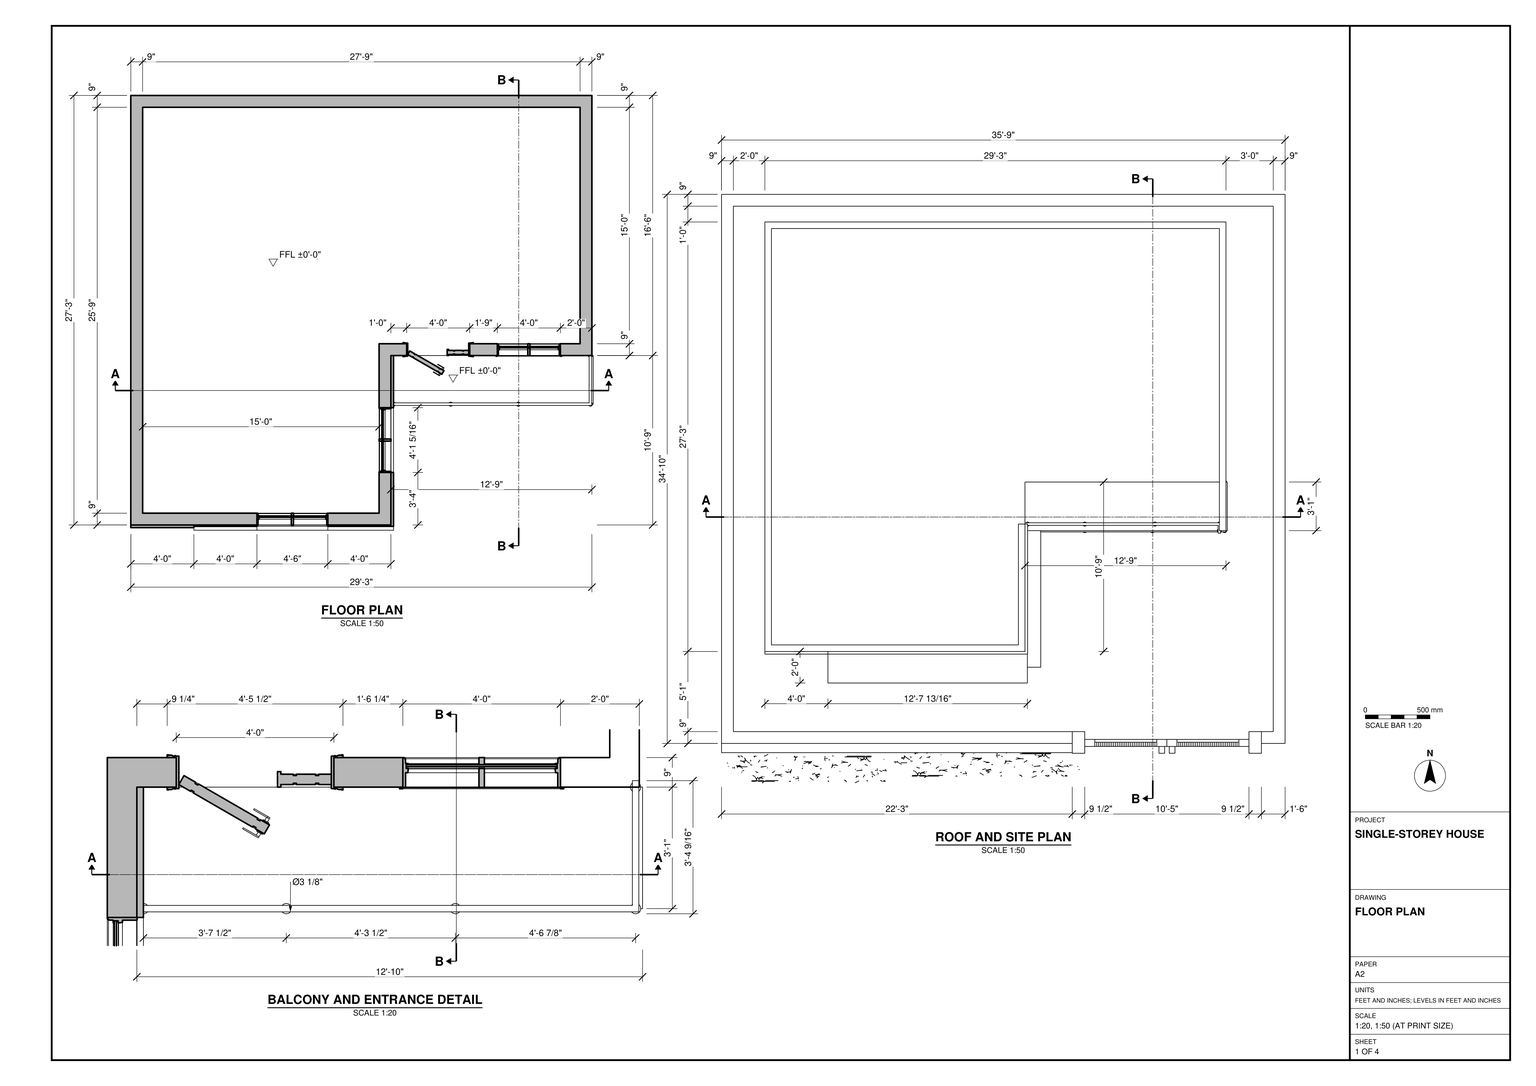
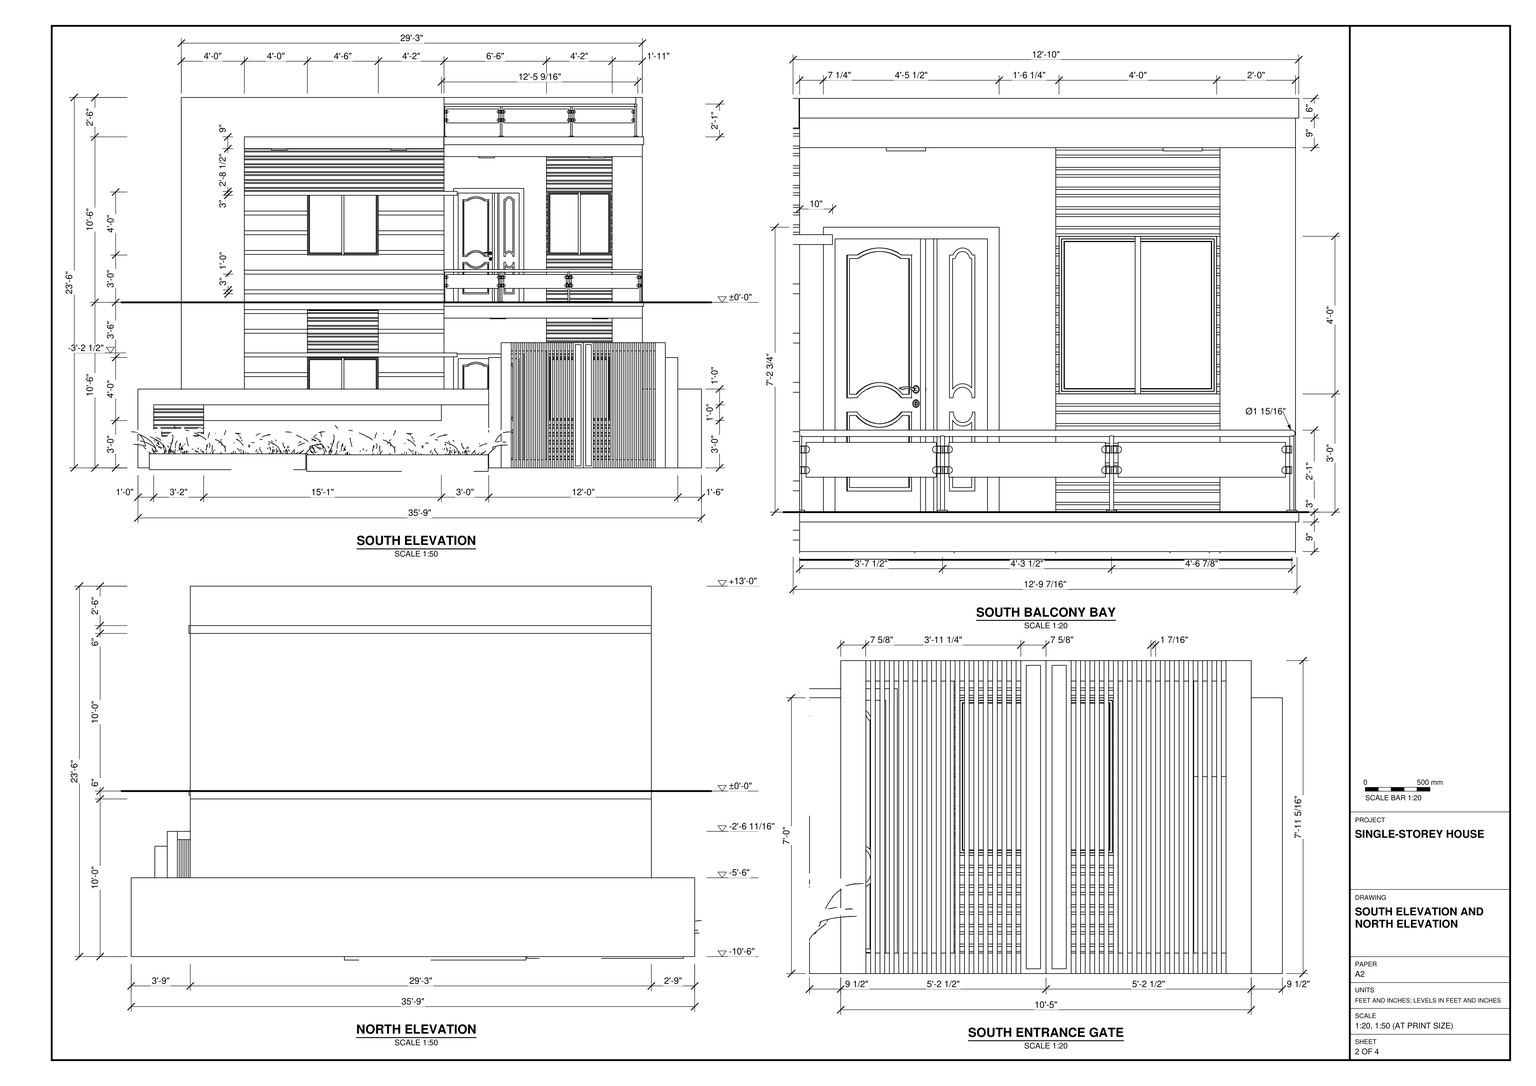
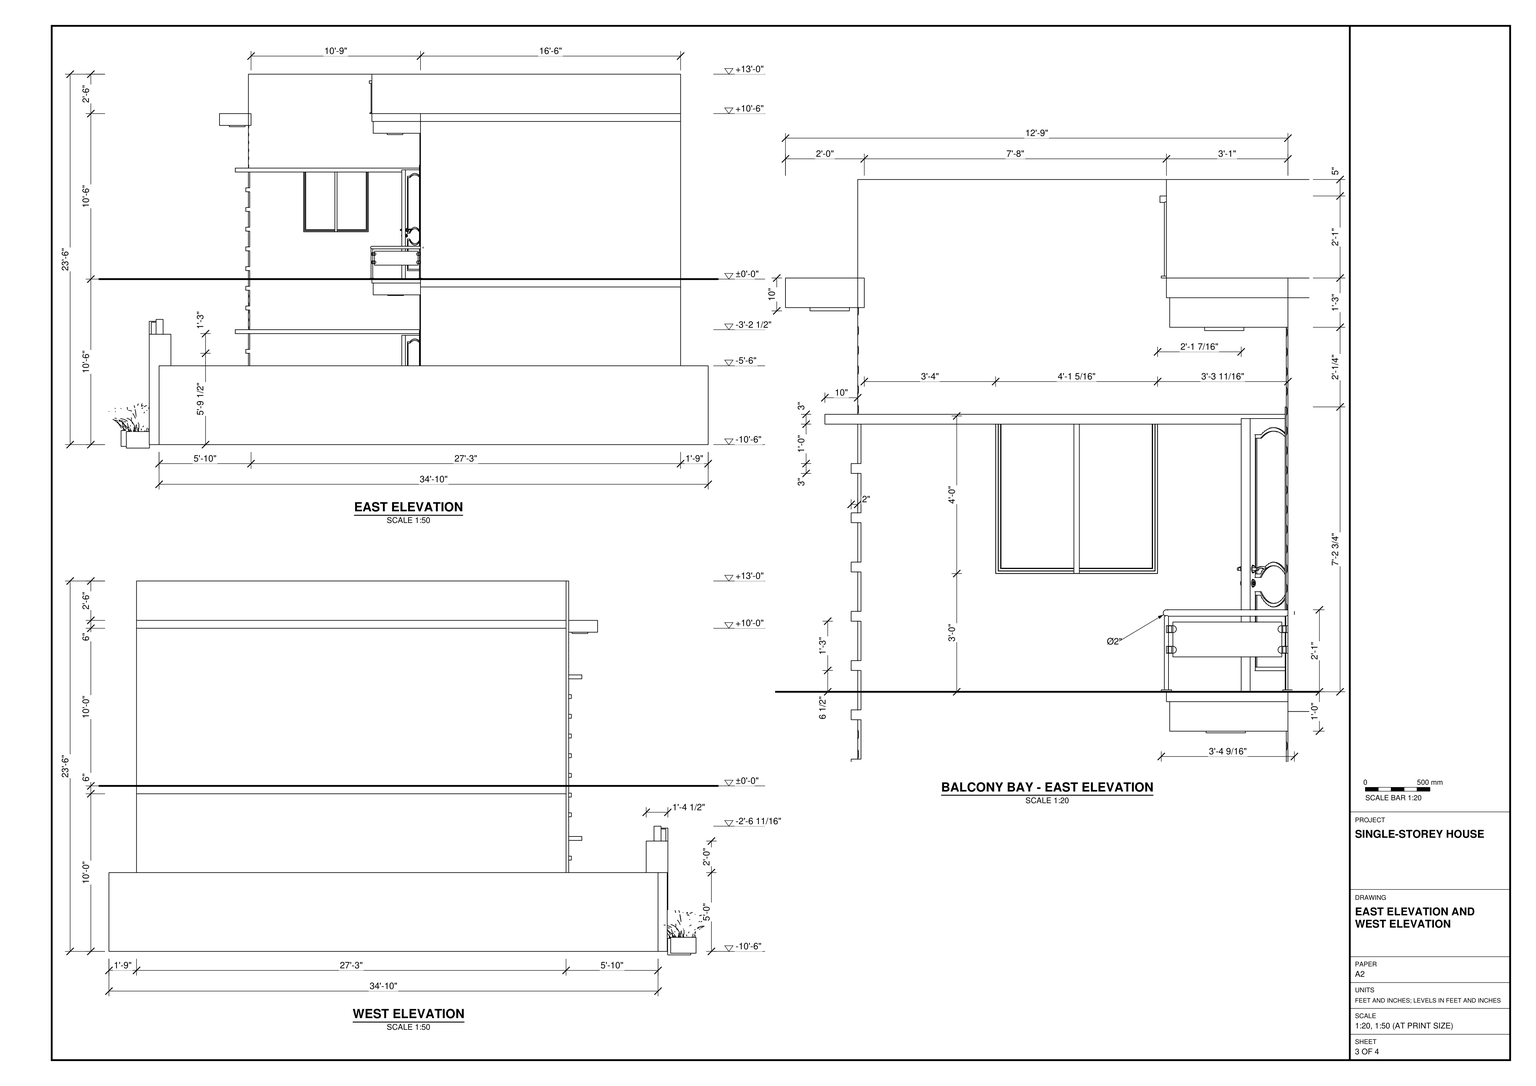
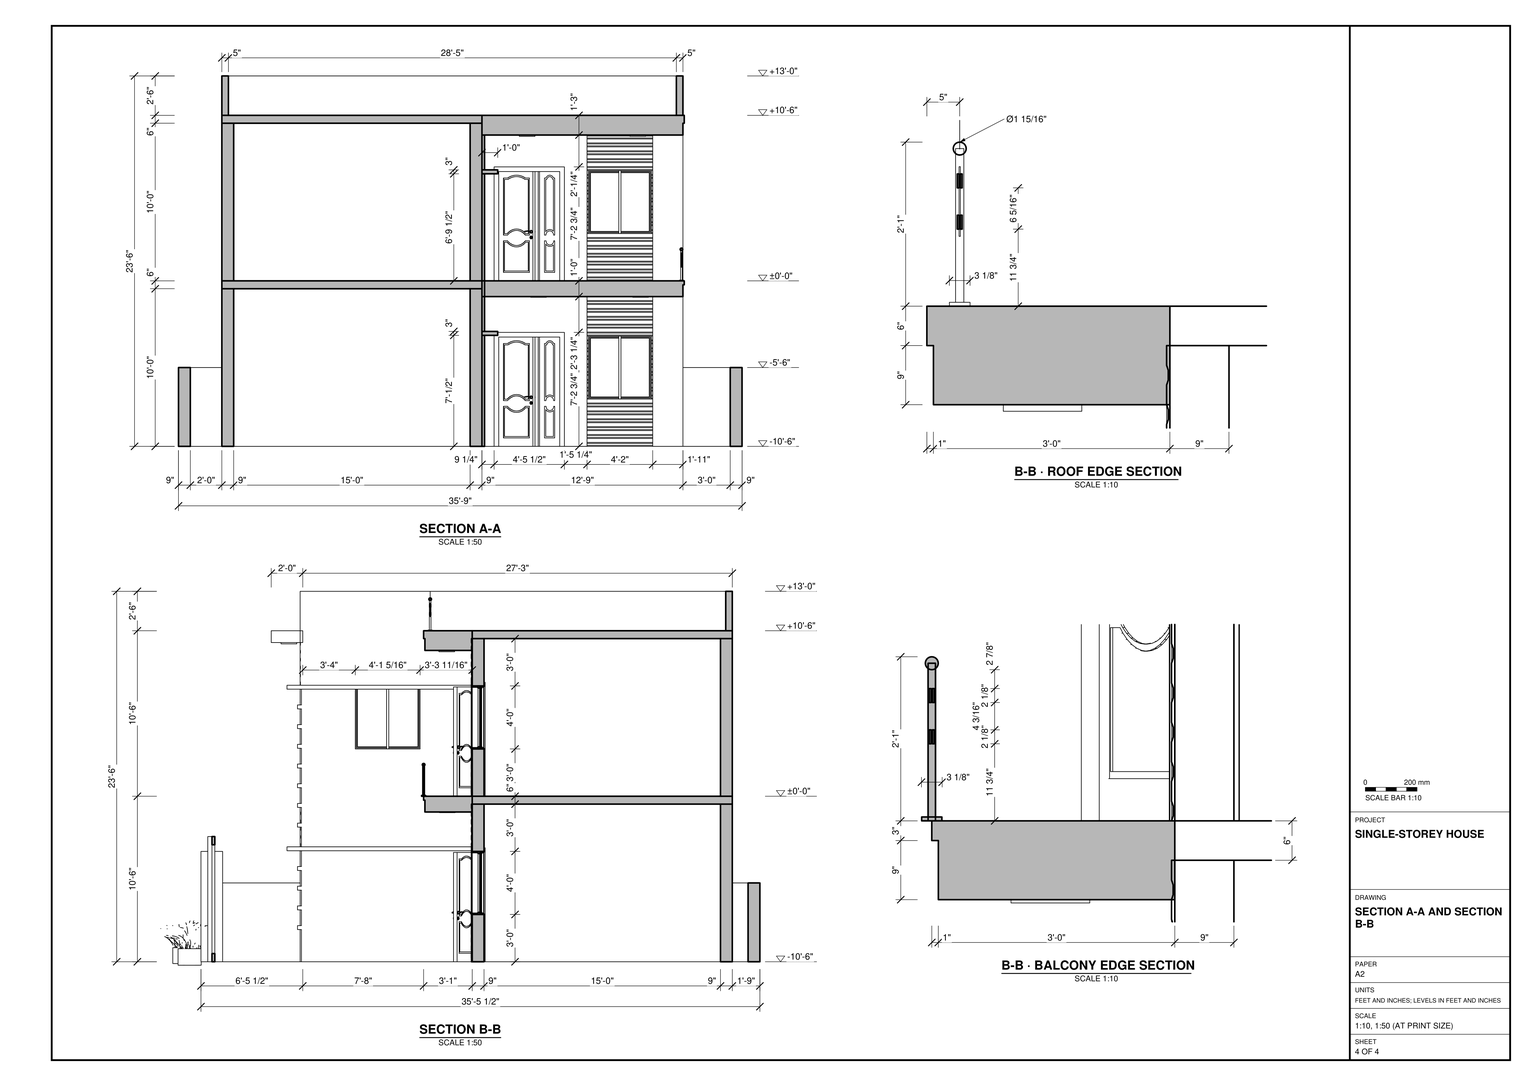
Build the house and its enclosing site in SketchUp from task_files/diagram_01.pdf. Work in feet and inches. The complete model, including the site elements, measures 36'-3 7/16" along X, 38'-1" along Y and 23'-8 11/16" along Z. Set the finished floor shown in plan to ±0'-0". Use the elevations to model the portion of the house visible below this datum as well as the walls and roof above it.

Lay out the 29'-3" by 27'-3" house footprint with the southeast corner recessed and the western wing extending toward the south boundary. Model the exterior walls at the drawn 9" thickness. In the recess, build the balcony slab, its front and return railings, the entrance door with its narrow side panel, and the adjacent framed window. Place the other windows in the projecting wing as shown. Match the horizontal bands on the south facade and the alignment of the openings above and below the floor datum. Form the flat roof with its parapets, projecting edges and railing above the balcony bay.

Follow the site plan for the boundary walls, south entrance gate and planted strip. Decor and loose items, including planting, may be any suitable library components. Keep walls, slabs, roof and other distinct assemblies in separate groups or components, keep each furniture or joinery piece separate, and use components for repeated parts. Save one SketchUp model as output_files/l_shaped_house_recessed_balcony_and_gated_site.skp.

# SketchUp Ruby script. Lengths in inches.
U = 1.inch
M = Sketchup.active_model
def pt(a) = Geom::Point3d.new(a.map { |v| v * U })
def face(e, loops, mat)
  f = e.add_face(loops[0].map { |a| pt(a) })
  loops[1..].each { |l| e.add_face(l.map { |a| pt(a) }).erase! }
  f.material = f.back_material = mat if mat
  f
end
# faces: each face lists its corners as indices into pts; further lists are holes
def faces(e, pts, list, mat = nil) = list.each { |f| face(e, (f[0].is_a?(Array) ? f : [f]).map { |l| l.map { |i| pts[i] } }, mat) }
# xy, xz, yz: faces in a plane at the given z, y or x. An outline is a flat list of corners, or four numbers for a rectangle; further outlines are holes
def ring(l) = l.size == 4 ? [[l[0], l[1]], [l[2], l[1]], [l[2], l[3]], [l[0], l[3]]] : l.each_slice(2).to_a
def flat(e, list, mat, &to3) = list.each { |f| face(e, (f[0].is_a?(Array) ? f : [f]).map { |l| ring(l).map { |u, v| to3.(u, v) } }, mat) }
def xy(e, z, list, mat = nil) = flat(e, list, mat) { |x, y| [x, y, z] }
def xz(e, y, list, mat = nil) = flat(e, list, mat) { |x, z| [x, y, z] }
def yz(e, x, list, mat = nil) = flat(e, list, mat) { |y, z| [x, y, z] }
def lines(e, pts, list) = list.each { |a, b| e.add_line(pt(pts[a]), pt(pts[b])) }
# prism: a flat outline (further loops are holes) pulled along v
def prism(e, loops, v, mat = nil)
  f = face(e, loops, mat); d = Geom::Vector3d.new(v.map { |x| x * U })
  f.pushpull(f.normal.samedirection?(d) ? d.length : -d.length)
end
def box(e, o, s, mat = nil) = prism(e, [[o, [o[0] + s[0], o[1], o[2]], [o[0] + s[0], o[1] + s[1], o[2]], [o[0], o[1] + s[1], o[2]]]], [0, 0, s[2]], mat)
def at(x, y, z, deg = 0) = Geom::Transformation.translation(pt([x, y, z])) * Geom::Transformation.rotation(ORIGIN, Z_AXIS, deg.degrees)
def axes(o, x, y, z) = Geom::Transformation.new([*x, 0, *y, 0, *z, 0, *pt(o).to_a, 1])
def part(name) = M.definitions.add(name)
# library, detail: a bought-in or finely detailed component or shape, given as its bounding box
def library(name, o, s) = part(name).tap { |d| box(d.entities, o, s) }
def detail(e, o, s) = box(e.add_group.entities, o, s)
def put(e, d, t, mat = nil) = e.add_instance(d, t).tap { |i| i.material = mat if mat }
def group(e, t, mat = nil) = e.add_group.tap { |g| g.transformation = t; g.material = mat if mat }.entities
root = M.entities
M.materials.add("[Color C02]").color = [255, 204, 153]
M.materials.add("[Color C07]").color = [153, 76, 0]
M.materials.add("[Color D02]").color = [255, 229, 153]
M.materials.add("[Color E04]").color = [255, 255, 50]
M.materials.add("[Granite Brown]").color = [126, 104, 91]
M.materials.add("[Granite Light Gray]").color = [149, 148, 144]
M.materials.add("[Metal Embossed]").color = [144, 144, 144]
M.materials.add("[Stone Brushed Khaki]").color = [226, 197, 133]
M.materials.add("[Wood Cherry Original]").color = [152, 86, 42]
c1 = library("Untitled (1)",[50.77,-2.25,0],[109.04,4.5625,95.3125])
c2 = library("Group\#1",[0,-0.35,0],[53.51,25.65,86.76])
c3 = library("Group\#3",[0,0,0],[48,9.07,48])
c4 = part("Group\#4")
prism(c4.entities,[[[0,0,0],[0,327,0],[351,327,0],[351,129,0],[198,129,0],[198,0,0]]],[0,0,6])
c5 = library("Group\#6",[0,0,0],[54,9.07,48])
c6 = library("Group\#8",[0,-0.5,0],[50,0.5,120])
c7 = library("Group\#15",[0,0,0],[9.07,49.3125,48])
c8 = part("Difference\#1")
xy(c8.entities,0,[[0,0,0,327,351,327,351,129,258,129,258,138,342,138,342,318,9,318,9,9,189,9,189,138,210,138,210,129,198,129,198,0]])
xy(c8.entities,36,[[96,0,150,9],[189,40,198,89.3125],[279,129,327,138]])
xy(c8.entities,84,[[96,0,150,9],[189,40,198,89.3125],[210,129,258,138],[279,129,327,138]])
xy(c8.entities,120,[[[0,0,198,0,198,129,351,129,351,327,0,327],[9,9,9,318,342,318,342,138,189,138,189,9]]])
xz(c8.entities,0,[[[0,0,198,120],[96,36,150,84]]])
xz(c8.entities,9,[[[9,0,189,120],[96,36,150,84]]])
xz(c8.entities,40,[[189,36,198,84]])
xz(c8.entities,89.3125,[[189,36,198,84]])
xz(c8.entities,129,[[[198,0,210,0,210,84,258,84,258,0,351,0,351,120,198,120],[279,36,327,84]]])
xz(c8.entities,138,[[[189,0,189,120,342,120,342,0,258,0,258,84,210,84,210,0],[279,36,327,84]]])
xz(c8.entities,318,[[9,0,342,120]])
xz(c8.entities,327,[[0,0,351,120]])
yz(c8.entities,0,[[0,0,327,120]])
yz(c8.entities,9,[[9,0,318,120]])
yz(c8.entities,96,[[0,36,9,84]])
yz(c8.entities,150,[[0,36,9,84]])
yz(c8.entities,189,[[[9,0,138,120],[40,36,89.3125,84]]])
yz(c8.entities,198,[[[0,0,129,120],[40,36,89.3125,84]]])
yz(c8.entities,210,[[129,0,138,84]])
yz(c8.entities,258,[[129,0,138,84]])
yz(c8.entities,279,[[129,36,138,84]])
yz(c8.entities,327,[[129,36,138,84]])
yz(c8.entities,342,[[138,0,318,120]])
yz(c8.entities,351,[[129,0,327,120]])
c9 = library("Group\#18",[0,0,0],[152,133,207.5])
c10 = part("Difference")
xy(c10.entities,0,[[0,0,0,327,351,327,351,129,258,129,258,138,342,138,342,318,9,318,9,9,189,9,189,138,210,138,210,129,198,129,198,0]])
xy(c10.entities,36,[[96,0,150,9],[279,129,327,138]])
xy(c10.entities,84,[[96,0,150,9],[210,129,258,138],[279,129,327,138]])
xy(c10.entities,120,[[[0,0,198,0,198,129,351,129,351,327,0,327],[9,9,9,318,342,318,342,138,189,138,189,9]]])
xz(c10.entities,0,[[[0,0,198,120],[96,36,150,84]]])
xz(c10.entities,9,[[[9,0,189,120],[96,36,150,84]]])
xz(c10.entities,129,[[[198,0,210,0,210,84,258,84,258,0,351,0,351,120,198,120],[279,36,327,84]]])
xz(c10.entities,138,[[[189,0,189,120,342,120,342,0,258,0,258,84,210,84,210,0],[279,36,327,84]]])
xz(c10.entities,318,[[9,0,342,120]])
xz(c10.entities,327,[[0,0,351,120]])
yz(c10.entities,0,[[0,0,327,120]])
yz(c10.entities,9,[[9,0,318,120]])
yz(c10.entities,96,[[0,36,9,84]])
yz(c10.entities,150,[[0,36,9,84]])
yz(c10.entities,189,[[9,0,138,120]])
yz(c10.entities,198,[[0,0,129,120]])
yz(c10.entities,210,[[129,0,138,84]])
yz(c10.entities,258,[[129,0,138,84]])
yz(c10.entities,279,[[129,36,138,84]])
yz(c10.entities,327,[[129,36,138,84]])
yz(c10.entities,342,[[138,0,318,120]])
yz(c10.entities,351,[[129,0,327,120]])
c11 = library("Group\#20",[0,0,0],[149.54,8.54,24.98])
c12 = library("Group\#21",[0,0,0],[153.42,40.54,24.98])
c13 = library("Group\#34",[0,0,0],[56.8,25.91,35.15])
put(root,c1,axes([218.3,5.21,0],[1.14636,0,0],[0,2.31507,0],[0,0,1]))
put(root,c2,at(240.24,191.05,0))
put(root,c3,at(360,215.5,36,180))
put(root,c4,at(33,77.5,120))
put(root,c5,at(183,86.5,36,180))
put(root,c5,at(183,86.5,162,180))
put(root,c2,at(240.24,191.05,126))
put(root,c3,at(360,215.5,162,180))
put(root,c6,at(311,206.5,126),"[Wood Cherry Original]")
g1 = group(root,at(81,65.5,84.5))
xy(g1,0,[[0,0,0,12,150,12,150,141,162,141,162,0]])
xy(g1,3,[[0,0,162,0,162,141,150,141,150,12,0,12]])
xz(g1,0,[[0,0,162,3]])
xz(g1,141,[[150,0,162,3]])
yz(g1,0,[[0,0,12,3]])
yz(g1,150,[[12,0,141,3]])
yz(g1,162,[[0,0,141,3]])
g2 = group(root,at(81,65.5,207.5))
xy(g2,0,[[0,0,0,12,150,12,150,141,162,141,162,0]])
xy(g2,3,[[0,0,162,0,162,141,150,141,150,12,0,12]])
xz(g2,0,[[0,0,162,3]])
xz(g2,141,[[150,0,162,3]])
yz(g2,0,[[0,0,12,3]])
yz(g2,150,[[12,0,141,3]])
yz(g2,162,[[0,0,141,3]])
g3 = group(root,at(129,75.5,87.5))
xy(g3,0,[[0,0,54,2]])
xy(g3,32.5,[[0,0,54,0.17]])
xy(g3,32.5,[[0,0.17,54,2]],"[Wood Cherry Original]")
xz(g3,0,[[0,3,54,6],[0,9,54,12],[0,15,54,18],[0,21,54,24],[0,27,54,30]],"[Wood Cherry Original]")
xz(g3,0.25,[[0,0.75,54,2.25],[0,6.75,54,8.25],[0,12.75,54,14.25],[0,18.75,54,20.25],[0,24.75,54,26.25],
  [0,30.75,54,32.25]],"[Wood Cherry Original]")
xz(g3,2,[[0,0,54,32.5]])
yz(g3,0,[[0,0,0,3,0.25,2.25,0.25,0.75],[0,6,0,9,0.25,8.25,0.25,6.75],[0,12,0,15,0.25,14.25,0.25,12.75],[0,18,0,21,0.25,20.25,0.25,18.75],[0,24,0,27,0.25,26.25,0.25,24.75],
  [0,30,0,32.5,0.17,32.5,0.25,32.25,0.25,30.75]])
yz(g3,0,[[0,0,0.25,0.75,0.25,2.25,0,3,0,6,0.25,6.75,0.25,8.25,0,9,0,12,0.25,12.75,0.25,14.25,0,15,0,18,0.25,18.75,0.25,20.25,0,21,0,24,0.25,24.75,0.25,26.25,0,27,0,30,0.25,30.75,0.25,32.25,0.17,32.5,2,32.5,2,0]],"[Wood Cherry Original]")
yz(g3,54,[[0,0,0.25,0.75,0.25,2.25,0,3],[0,6,0.25,6.75,0.25,8.25,0,9],[0,12,0.25,12.75,0.25,14.25,0,15],[0,18,0.25,18.75,0.25,20.25,0,21],[0,24,0.25,24.75,0.25,26.25,0,27],
  [0,30,0.25,30.75,0.25,32.25,0.17,32.5,0,32.5]])
yz(g3,54,[[0,0,2,0,2,32.5,0.17,32.5,0.25,32.25,0.25,30.75,0,30,0,27,0.25,26.25,0.25,24.75,0,24,0,21,0.25,20.25,0.25,18.75,0,18,0,15,0.25,14.25,0.25,12.75,0,12,0,9,0.25,8.25,0.25,6.75,0,6,0,3,0.25,2.25,0.25,0.75]],"[Wood Cherry Original]")
p = [[54,0.25,0.75],[0,0.25,0.75],[0,0,0],[54,0,0],[54,0,3],[0,0,3],
  [0,0.25,2.25],[54,0.25,2.25],[54,0.25,6.75],[0,0.25,6.75],[0,0,6],[54,0,6],
  [54,0,9],[0,0,9],[0,0.25,8.25],[54,0.25,8.25],[54,0.25,12.75],[0,0.25,12.75],
  [0,0,12],[54,0,12],[54,0,15],[0,0,15],[0,0.25,14.25],[54,0.25,14.25],
  [54,0.25,18.75],[0,0.25,18.75],[0,0,18],[54,0,18],[54,0,21],[0,0,21],
  [0,0.25,20.25],[54,0.25,20.25],[54,0.25,24.75],[0,0.25,24.75],[0,0,24],[54,0,24],
  [54,0,27],[0,0,27],[0,0.25,26.25],[54,0.25,26.25],[54,0.25,30.75],[0,0.25,30.75],
  [0,0,30],[54,0,30],[0,0.25,32.25],[54,0.25,32.25],[54,0.17,32.5],[0,0.17,32.5]]
faces(g3,p,[[0,1,2,3],[4,5,6,7],[8,9,10,11],[12,13,14,15],[16,17,18,19],[20,21,22,23],[24,25,26,27],[28,29,30,31],
  [32,33,34,35],[36,37,38,39],[40,41,42,43]],"[Wood Cherry Original]")
faces(g3,p,[[44,45,46,47]])
put(root,c6,at(311,206.5,0),"[Wood Cherry Original]")
g4 = group(root,at(231,169.5,113.5))
xy(g4,0,[[43.26,12.0625,41.7,12.22,40.24,12.77,38.97,13.68,37.97,14.89,37.33,16.32,37.07,17.87,37.23,19.42,37.78,20.89,38.69,22.16,39.9,23.16,41.33,23.8,42.875,24.06,44.43,23.9,45.9,23.35,47.17,22.4375,48.17,21.23,48.8125,19.8,49.07,18.25,48.91,16.7,48.36,15.23,47.45,13.96,46.24,12.96,44.81,12.32],[120.57,12.0625,119.02,12.32,117.6,12.96,116.39,13.96,115.47,15.23,114.92,16.7,114.77,18.25,115.02,19.8,115.67,21.23,116.66,22.4375,117.93,23.35,119.4,23.9,120.96,24.06,122.5,23.8,123.93,23.16,125.14,22.16,126.05,20.89,126.61,19.42,126.76,17.87,126.51,16.32,125.86,14.89,124.87,13.68,123.59,12.77,122.13,12.22]],"[Color E04]")
xy(g4,0.5,[[[0,1,153,37],[120.57,12.0625,122.13,12.22,123.59,12.77,124.87,13.68,125.86,14.89,126.51,16.32,126.76,17.87,126.61,19.42,126.05,20.89,125.14,22.16,123.93,23.16,122.5,23.8,120.96,24.06,119.4,23.9,117.93,23.35,116.66,22.4375,115.67,21.23,115.02,19.8,114.77,18.25,114.92,16.7,115.47,15.23,116.39,13.96,117.6,12.96,119.02,12.32],[43.26,12.0625,44.81,12.32,46.24,12.96,47.45,13.96,48.36,15.23,48.91,16.7,49.07,18.25,48.8125,19.8,48.17,21.23,47.17,22.4375,45.9,23.35,44.43,23.9,42.875,24.06,41.33,23.8,39.9,23.16,38.69,22.16,37.78,20.89,37.23,19.42,37.07,17.87,37.33,16.32,37.97,14.89,38.97,13.68,40.24,12.77,41.7,12.22]]],"[Granite Light Gray]")
xy(g4,9.5,[[0,0,0,1,153,1,153,37,154,37,154,0]])
xy(g4,12.5,[[0,0,154,37]])
xz(g4,0,[[0,9.5,154,12.5]])
xz(g4,1,[[0,0.5,153,9.5]],"[Granite Light Gray]")
xz(g4,37,[[0,0.5,0,12.5,154,12.5,154,9.5,153,9.5,153,0.5]])
yz(g4,0,[[1,0.5,1,9.5,0,9.5,0,12.5,37,12.5,37,0.5]])
yz(g4,153,[[1,0.5,37,9.5]],"[Granite Light Gray]")
yz(g4,154,[[0,9.5,37,12.5]])
p = [[43.26,12.0625,0.5],[41.7,12.22,0.5],[41.7,12.22,0],[43.26,12.0625,0],[44.81,12.32,0.5],[44.81,12.32,0],
  [120.57,12.0625,0.5],[119.02,12.32,0.5],[119.02,12.32,0],[120.57,12.0625,0],[122.13,12.22,0.5],[122.13,12.22,0],
  [40.24,12.77,0.5],[40.24,12.77,0],[123.59,12.77,0.5],[123.59,12.77,0],[46.24,12.96,0.5],[46.24,12.96,0],
  [117.6,12.96,0.5],[117.6,12.96,0],[38.97,13.68,0.5],[38.97,13.68,0],[124.87,13.68,0.5],[124.87,13.68,0],
  [47.45,13.96,0.5],[47.45,13.96,0],[116.39,13.96,0.5],[116.39,13.96,0],[37.97,14.89,0.5],[37.97,14.89,0],
  [125.86,14.89,0.5],[125.86,14.89,0],[48.36,15.23,0.5],[48.36,15.23,0],[115.47,15.23,0.5],[115.47,15.23,0],
  [37.33,16.32,0.5],[37.33,16.32,0],[126.51,16.32,0.5],[126.51,16.32,0],[48.91,16.7,0.5],[48.91,16.7,0],
  [114.92,16.7,0.5],[114.92,16.7,0],[37.07,17.87,0.5],[37.07,17.87,0],[126.76,17.87,0.5],[126.76,17.87,0],
  [49.07,18.25,0.5],[49.07,18.25,0],[114.77,18.25,0.5],[114.77,18.25,0],[37.23,19.42,0.5],[37.23,19.42,0],
  [126.61,19.42,0.5],[126.61,19.42,0],[48.8125,19.8,0.5],[48.8125,19.8,0],[115.02,19.8,0.5],[115.02,19.8,0],
  [37.78,20.89,0.5],[37.78,20.89,0],[126.05,20.89,0.5],[126.05,20.89,0],[48.17,21.23,0.5],[48.17,21.23,0],
  [115.67,21.23,0.5],[115.67,21.23,0],[38.69,22.16,0.5],[38.69,22.16,0],[125.14,22.16,0.5],[125.14,22.16,0],
  [47.17,22.4375,0.5],[47.17,22.4375,0],[116.66,22.4375,0.5],[116.66,22.4375,0],[39.9,23.16,0.5],[39.9,23.16,0],
  [123.93,23.16,0.5],[123.93,23.16,0],[45.9,23.35,0.5],[45.9,23.35,0],[117.93,23.35,0.5],[117.93,23.35,0],
  [41.33,23.8,0.5],[41.33,23.8,0],[122.5,23.8,0.5],[122.5,23.8,0],[44.43,23.9,0.5],[44.43,23.9,0],
  [119.4,23.9,0.5],[119.4,23.9,0],[42.875,24.06,0.5],[42.875,24.06,0],[120.96,24.06,0.5],[120.96,24.06,0]]
faces(g4,p,[[0,1,2,3],[4,0,3,5],[6,7,8,9],[10,6,9,11],[1,12,13,2],[14,10,11,15],[16,4,5,17],[7,18,19,8],
  [12,20,21,13],[22,14,15,23],[24,16,17,25],[18,26,27,19],[20,28,29,21],[30,22,23,31],[32,24,25,33],[26,34,35,27],
  [28,36,37,29],[38,30,31,39],[40,32,33,41],[34,42,43,35],[36,44,45,37],[46,38,39,47],[48,40,41,49],[42,50,51,43],
  [44,52,53,45],[54,46,47,55],[56,48,49,57],[50,58,59,51],[52,60,61,53],[62,54,55,63],[64,56,57,65],[58,66,67,59],
  [60,68,69,61],[70,62,63,71],[72,64,65,73],[66,74,75,67],[68,76,77,69],[78,70,71,79],[80,72,73,81],[74,82,83,75],
  [76,84,85,77],[86,78,79,87],[88,80,81,89],[82,90,91,83],[84,92,93,85],[94,86,87,95],[92,88,89,93],[90,94,95,91]],"[Color E04]")
g5 = group(root,at(81,53.5,242))
g6 = group(g5,at(0,0,0))
xy(g6,0,[[26.54,7.46,24.99,7.67,23.54,8.27,22.3,9.22,21.35,10.46,20.75,11.91,20.54,13.46,20.75,15.02,21.35,16.46,22.3,17.7,23.54,18.66,24.99,19.26,26.54,19.46,28.1,19.26,29.54,18.66,30.79,17.7,31.74,16.46,32.34,15.02,32.54,13.46,32.34,11.91,31.74,10.46,30.79,9.22,29.54,8.27,28.1,7.67],[117.54,7.46,115.99,7.67,114.54,8.27,113.3,9.22,112.35,10.46,111.75,11.91,111.54,13.46,111.75,15.02,112.35,16.46,113.3,17.7,114.54,18.66,115.99,19.26,117.54,19.46,119.1,19.26,120.54,18.66,121.79,17.7,122.74,16.46,123.34,15.02,123.54,13.46,123.34,11.91,122.74,10.46,121.79,9.22,120.54,8.27,119.1,7.67]],"[Color E04]")
xy(g6,1,[[[0,0,151.8125,24],[26.54,7.46,28.1,7.67,29.54,8.27,30.79,9.22,31.74,10.46,32.34,11.91,32.54,13.46,32.34,15.02,31.74,16.46,30.79,17.7,29.54,18.66,28.1,19.26,26.54,19.46,24.99,19.26,23.54,18.66,22.3,17.7,21.35,16.46,20.75,15.02,20.54,13.46,20.75,11.91,21.35,10.46,22.3,9.22,23.54,8.27,24.99,7.67],[117.54,7.46,119.1,7.67,120.54,8.27,121.79,9.22,122.74,10.46,123.34,11.91,123.54,13.46,123.34,15.02,122.74,16.46,121.79,17.7,120.54,18.66,119.1,19.26,117.54,19.46,115.99,19.26,114.54,18.66,113.3,17.7,112.35,16.46,111.75,15.02,111.54,13.46,111.75,11.91,112.35,10.46,113.3,9.22,114.54,8.27,115.99,7.67]]])
xy(g6,10,[[0,0,151.8125,24]])
xz(g6,0,[[0,1,151.8125,10]])
xz(g6,24,[[0,1,151.8125,10]])
yz(g6,0,[[0,1,24,10]])
yz(g6,151.8125,[[0,1,24,10]])
p = [[26.54,7.46,1],[24.99,7.67,1],[24.99,7.67,0],[26.54,7.46,0],[28.1,7.67,1],[28.1,7.67,0],
  [117.54,7.46,1],[115.99,7.67,1],[115.99,7.67,0],[117.54,7.46,0],[119.1,7.67,1],[119.1,7.67,0],
  [23.54,8.27,1],[23.54,8.27,0],[29.54,8.27,1],[29.54,8.27,0],[114.54,8.27,1],[114.54,8.27,0],
  [120.54,8.27,1],[120.54,8.27,0],[22.3,9.22,1],[22.3,9.22,0],[30.79,9.22,1],[30.79,9.22,0],
  [113.3,9.22,1],[113.3,9.22,0],[121.79,9.22,1],[121.79,9.22,0],[21.35,10.46,1],[21.35,10.46,0],
  [31.74,10.46,1],[31.74,10.46,0],[112.35,10.46,1],[112.35,10.46,0],[122.74,10.46,1],[122.74,10.46,0],
  [20.75,11.91,1],[20.75,11.91,0],[32.34,11.91,1],[32.34,11.91,0],[111.75,11.91,1],[111.75,11.91,0],
  [123.34,11.91,1],[123.34,11.91,0],[20.54,13.46,1],[20.54,13.46,0],[32.54,13.46,1],[32.54,13.46,0],
  [111.54,13.46,1],[111.54,13.46,0],[123.54,13.46,1],[123.54,13.46,0],[20.75,15.02,1],[20.75,15.02,0],
  [32.34,15.02,1],[32.34,15.02,0],[111.75,15.02,1],[111.75,15.02,0],[123.34,15.02,1],[123.34,15.02,0],
  [21.35,16.46,1],[21.35,16.46,0],[31.74,16.46,1],[31.74,16.46,0],[112.35,16.46,1],[112.35,16.46,0],
  [122.74,16.46,1],[122.74,16.46,0],[22.3,17.7,1],[22.3,17.7,0],[30.79,17.7,1],[30.79,17.7,0],
  [113.3,17.7,1],[113.3,17.7,0],[121.79,17.7,1],[121.79,17.7,0],[23.54,18.66,1],[23.54,18.66,0],
  [29.54,18.66,1],[29.54,18.66,0],[114.54,18.66,1],[114.54,18.66,0],[120.54,18.66,1],[120.54,18.66,0],
  [24.99,19.26,1],[24.99,19.26,0],[28.1,19.26,1],[28.1,19.26,0],[115.99,19.26,1],[115.99,19.26,0],
  [119.1,19.26,1],[119.1,19.26,0],[26.54,19.46,1],[26.54,19.46,0],[117.54,19.46,1],[117.54,19.46,0]]
faces(g6,p,[[0,1,2,3],[4,0,3,5],[6,7,8,9],[10,6,9,11],[1,12,13,2],[14,4,5,15],[7,16,17,8],[18,10,11,19],
  [12,20,21,13],[22,14,15,23],[16,24,25,17],[26,18,19,27],[20,28,29,21],[30,22,23,31],[24,32,33,25],[34,26,27,35],
  [28,36,37,29],[38,30,31,39],[32,40,41,33],[42,34,35,43],[36,44,45,37],[46,38,39,47],[40,48,49,41],[50,42,43,51],
  [44,52,53,45],[54,46,47,55],[48,56,57,49],[58,50,51,59],[52,60,61,53],[62,54,55,63],[56,64,65,57],[66,58,59,67],
  [60,68,69,61],[70,62,63,71],[64,72,73,65],[74,66,67,75],[68,76,77,69],[78,70,71,79],[72,80,81,73],[82,74,75,83],
  [76,84,85,77],[86,78,79,87],[80,88,89,81],[90,82,83,91],[84,92,93,85],[92,86,87,93],[88,94,95,89],[94,90,91,95]],"[Color E04]")
put(root,c7,at(231.07,166.8125,162,180))
g7 = group(root,at(231,169.5,236))
xy(g7,0,[[34.91,11.63,33.35,11.7,31.85,12.17,30.53,13.01,29.47,14.16,28.75,15.55,28.41,17.08,28.47,18.65,28.94,20.14,29.78,21.46,30.93,22.52,32.32,23.25,33.85,23.59,35.42,23.52,36.91,23.05,38.23,22.21,39.29,21.06,40.02,19.67,40.36,18.14,40.29,16.58,39.82,15.08,38.98,13.76,37.83,12.7,36.44,11.98],[118.09,11.63,116.56,11.98,115.17,12.7,114.02,13.76,113.18,15.08,112.71,16.58,112.64,18.14,112.98,19.67,113.71,21.06,114.77,22.21,116.09,23.05,117.58,23.52,119.15,23.59,120.68,23.25,122.07,22.52,123.22,21.46,124.06,20.14,124.53,18.65,124.59,17.08,124.25,15.55,123.53,14.16,122.47,13.01,121.15,12.17,119.65,11.7]],"[Color E04]")
xy(g7,1,[[[0,1,153,37],[118.09,11.63,119.65,11.7,121.15,12.17,122.47,13.01,123.53,14.16,124.25,15.55,124.59,17.08,124.53,18.65,124.06,20.14,123.22,21.46,122.07,22.52,120.68,23.25,119.15,23.59,117.58,23.52,116.09,23.05,114.77,22.21,113.71,21.06,112.98,19.67,112.64,18.14,112.71,16.58,113.18,15.08,114.02,13.76,115.17,12.7,116.56,11.98],[34.91,11.63,36.44,11.98,37.83,12.7,38.98,13.76,39.82,15.08,40.29,16.58,40.36,18.14,40.02,19.67,39.29,21.06,38.23,22.21,36.91,23.05,35.42,23.52,33.85,23.59,32.32,23.25,30.93,22.52,29.78,21.46,28.94,20.14,28.47,18.65,28.41,17.08,28.75,15.55,29.47,14.16,30.53,13.01,31.85,12.17,33.35,11.7]]],"[Granite Light Gray]")
xy(g7,10,[[0,0,0,1,153,1,153,37,154,37,154,0]])
xy(g7,16,[[0,0,154,37]])
xz(g7,0,[[0,10,154,16]])
xz(g7,1,[[0,1,153,10]],"[Granite Light Gray]")
xz(g7,37,[[0,1,0,16,154,16,154,10,153,10,153,1]])
yz(g7,0,[[1,1,1,10,0,10,0,16,37,16,37,1]])
yz(g7,153,[[1,1,37,10]],"[Granite Light Gray]")
yz(g7,154,[[0,10,37,16]])
p = [[34.91,11.63,1],[33.35,11.7,1],[33.35,11.7,0],[34.91,11.63,0],[36.44,11.98,1],[36.44,11.98,0],
  [118.09,11.63,1],[116.56,11.98,1],[116.56,11.98,0],[118.09,11.63,0],[119.65,11.7,1],[119.65,11.7,0],
  [31.85,12.17,1],[31.85,12.17,0],[121.15,12.17,1],[121.15,12.17,0],[37.83,12.7,1],[37.83,12.7,0],
  [115.17,12.7,1],[115.17,12.7,0],[30.53,13.01,1],[30.53,13.01,0],[122.47,13.01,1],[122.47,13.01,0],
  [38.98,13.76,1],[38.98,13.76,0],[114.02,13.76,1],[114.02,13.76,0],[29.47,14.16,1],[29.47,14.16,0],
  [123.53,14.16,1],[123.53,14.16,0],[39.82,15.08,1],[39.82,15.08,0],[113.18,15.08,1],[113.18,15.08,0],
  [28.75,15.55,1],[28.75,15.55,0],[124.25,15.55,1],[124.25,15.55,0],[40.29,16.58,1],[40.29,16.58,0],
  [112.71,16.58,1],[112.71,16.58,0],[28.41,17.08,1],[28.41,17.08,0],[124.59,17.08,1],[124.59,17.08,0],
  [40.36,18.14,1],[40.36,18.14,0],[112.64,18.14,1],[112.64,18.14,0],[28.47,18.65,1],[28.47,18.65,0],
  [124.53,18.65,1],[124.53,18.65,0],[40.02,19.67,1],[40.02,19.67,0],[112.98,19.67,1],[112.98,19.67,0],
  [28.94,20.14,1],[28.94,20.14,0],[124.06,20.14,1],[124.06,20.14,0],[39.29,21.06,1],[39.29,21.06,0],
  [113.71,21.06,1],[113.71,21.06,0],[29.78,21.46,1],[29.78,21.46,0],[123.22,21.46,1],[123.22,21.46,0],
  [38.23,22.21,1],[38.23,22.21,0],[114.77,22.21,1],[114.77,22.21,0],[30.93,22.52,1],[30.93,22.52,0],
  [122.07,22.52,1],[122.07,22.52,0],[36.91,23.05,1],[36.91,23.05,0],[116.09,23.05,1],[116.09,23.05,0],
  [32.32,23.25,1],[32.32,23.25,0],[120.68,23.25,1],[120.68,23.25,0],[35.42,23.52,1],[35.42,23.52,0],
  [117.58,23.52,1],[117.58,23.52,0],[33.85,23.59,1],[33.85,23.59,0],[119.15,23.59,1],[119.15,23.59,0]]
faces(g7,p,[[0,1,2,3],[4,0,3,5],[6,7,8,9],[10,6,9,11],[1,12,13,2],[14,10,11,15],[16,4,5,17],[7,18,19,8],
  [12,20,21,13],[22,14,15,23],[24,16,17,25],[18,26,27,19],[20,28,29,21],[30,22,23,31],[32,24,25,33],[26,34,35,27],
  [28,36,37,29],[38,30,31,39],[40,32,33,41],[34,42,43,35],[36,44,45,37],[46,38,39,47],[48,40,41,49],[42,50,51,43],
  [44,52,53,45],[54,46,47,55],[56,48,49,57],[50,58,59,51],[52,60,61,53],[62,54,55,63],[64,56,57,65],[58,66,67,59],
  [60,68,69,61],[70,62,63,71],[72,64,65,73],[66,74,75,67],[68,76,77,69],[78,70,71,79],[80,72,73,81],[74,82,83,75],
  [76,84,85,77],[86,78,79,87],[88,80,81,89],[82,90,91,83],[84,92,93,85],[94,86,87,95],[92,88,89,93],[90,94,95,91]],"[Color E04]")
g8 = group(root,at(33,77.5,252),"[Color D02]")
xy(g8,0,[[5,5,193,5,193,97,198,97,198,92,346,92,346,322,5,322]])
xy(g8,30,[[0,0,198,0,198,97,193,97,193,5,5,5,5,322,346,322,346,92,351,92,351,327,0,327]])
xz(g8,0,[[0,0,198,30]])
xz(g8,5,[[5,0,193,30]])
xz(g8,92,[[346,0,351,30]])
xz(g8,97,[[193,0,198,30]])
xz(g8,322,[[5,0,346,30]])
xz(g8,327,[[0,0,351,30]])
yz(g8,0,[[0,0,327,30]])
yz(g8,5,[[5,0,322,30]])
yz(g8,193,[[5,0,97,30]])
yz(g8,198,[[0,0,97,30]])
yz(g8,346,[[92,0,322,30]])
yz(g8,351,[[92,0,327,30]])
put(root,c4,at(33,77.5,246),"[Color D02]")
put(root,c8,at(33,77.5,126),"[Stone Brushed Khaki]")
g9 = group(root,at(33,75.5,0))
xy(g9,0,[[0,0,48,2]])
xy(g9,210.5,[[48,0,198,2],[198,0,200,131]])
xy(g9,237,[[198,95,200,131]])
xy(g9,246,[[198,94,200,95]])
xy(g9,252,[[198,94,200,99]])
xy(g9,282,[[0,0,48,2],[48,0,200,0,200,99,198,99,198,2,48,2]])
xz(g9,0,[[48,213.5,200,216.5],[48,219.5,200,222.5],[48,225.5,200,228.5],[48,231.5,200,234.5],[48,237.5,200,240.5]],"[Color C07]")
xz(g9,0,[[0,0,48,0,48,243,200,243,200,282,0,282]],"[Metal Embossed]")
xz(g9,0.25,[[48,211.25,200,212.75],[48,217.25,200,218.75],[48,223.25,200,224.75],[48,229.25,200,230.75],[48,235.25,200,236.75],
  [48,241.25,200,242.75]],"[Color C07]")
xz(g9,2,[[0,0,48,282]])
xz(g9,94,[[198,246,200,252]])
xz(g9,95,[[198,237,200,246]])
xz(g9,99,[[198,252,200,282]])
xz(g9,131,[[198,210.5,200,237]])
yz(g9,0,[[0,0,2,282]])
yz(g9,48,[[0,0,2,210.5],[0,243,2,252]])
yz(g9,200,[[0,210.5,0.25,211.25,0.25,212.75,0,213.5],[0,216.5,0.25,217.25,0.25,218.75,0,219.5],[0,222.5,0.25,223.25,0.25,224.75,0,225.5],[0,228.5,0.25,229.25,0.25,230.75,0,231.5],[0,234.5,0.25,235.25,0.25,236.75,0,237.5]])
yz(g9,200,[[0,210.5,131,210.5,131,237,95,237,95,246,94,246,94,252,99,252,99,282,0,282,0,237.5,0.25,236.75,0.25,235.25,0,234.5,0,231.5,0.25,230.75,0.25,229.25,0,228.5,0,225.5,0.25,224.75,0.25,223.25,0,222.5,0,219.5,0.25,218.75,0.25,217.25,0,216.5,0,213.5,0.25,212.75,0.25,211.25]],"[Metal Embossed]")
p = [[198,0,210.5],[200,0,210.5],[200,0.25,211.25],[48,0.25,211.25],[48,0,210.5],[48,0.25,212.75],
  [200,0.25,212.75],[200,0,213.5],[48,0,213.5],[48,0,216.5],[200,0,216.5],[200,0.25,217.25],
  [48,0.25,217.25],[48,0.25,218.75],[200,0.25,218.75],[200,0,219.5],[48,0,219.5],[48,0,222.5],
  [200,0,222.5],[200,0.25,223.25],[48,0.25,223.25],[48,0.25,224.75],[200,0.25,224.75],[200,0,225.5],
  [48,0,225.5],[48,0,228.5],[200,0,228.5],[200,0.25,229.25],[48,0.25,229.25],[48,0.25,230.75],
  [200,0.25,230.75],[200,0,231.5],[48,0,231.5],[48,0,234.5],[200,0,234.5],[200,0.25,235.25],
  [48,0.25,235.25],[48,0.25,236.75],[200,0.25,236.75],[200,0,237.5],[48,0,237.5],[48,0,240.5],
  [200,0,240.5],[200,0.25,241.25],[48,0.25,241.25],[48,0.25,242.75],[200,0.25,242.75],[200,0.17,243],
  [48,0.17,243],[198,0,252],[48,0,252],[198,94,252]]
faces(g9,p,[[0,1,2,3,4],[5,6,7,8],[9,10,11,12],[13,14,15,16],[17,18,19,20],[21,22,23,24],[25,26,27,28],[29,30,31,32],
  [33,34,35,36],[37,38,39,40],[41,42,43,44],[45,46,47,48]],"[Color C07]")
lines(g9,p,[[49,50],[51,49]])
put(root,c9,at(81,73.5,0))
put(root,c10,at(33,77.5,0),"[Stone Brushed Khaki]")
put(root,c11,at(231.03,167.53,252))
put(root,c12,at(231.03,167.93,126))
g10 = group(root,at(0,7.5,0),"[Color C02]")
prism(g10,[[[411,9,0],[420,9,0],[420,409,0],[9,409,0],[9,9,0],[267,9,0],[267,0,0],[0,0,0],[0,418,0],[429,418,0],[429,0,0],[411,0,0]]],[0,0,60])
g11 = group(root,at(267,0,0),"[Granite Brown]")
box(g11,[0,0,0],[9.5,16.5,84])
g12 = group(root,at(401.5,0,0),"[Granite Brown]")
box(g12,[0,0,0],[9.5,16.5,84])
g13 = group(root,at(0,1.5,0),"[Color D02]")
prism(g13,[[[0,6,0],[0,6,60],[267,6,60],[267,6,48],[12,6,48],[12,6,0]]],[0,-7,0])
g14 = group(root,at(12,3.5,0),"[Color C07]")
xy(g14,0,[[0,0,38.03,4]])
xy(g14,48,[[0,0,38.03,4]])
xz(g14,0,[[0,3,38.03,6],[0,9,38.03,12],[0,15,38.03,18],[0,21,38.03,24],[0,27,38.03,30],
  [0,33,38.03,36],[0,39,38.03,42],[0,45,38.03,48]])
xz(g14,0.25,[[0,0.75,38.03,2.25],[0,6.75,38.03,8.25],[0,12.75,38.03,14.25],[0,18.75,38.03,20.25],[0,24.75,38.03,26.25],
  [0,30.75,38.03,32.25],[0,36.75,38.03,38.25],[0,42.75,38.03,44.25]])
xz(g14,4,[[0,0,38.03,48]])
yz(g14,0,[[0,0,0,3,0.25,2.25,0.25,0.75],[0,0,0.25,0.75,0.25,2.25,0,3,0,6,0.25,6.75,0.25,8.25,0,9,0,12,0.25,12.75,0.25,14.25,0,15,0,18,0.25,18.75,0.25,20.25,0,21,0,24,0.25,24.75,0.25,26.25,0,27,0,30,0.25,30.75,0.25,32.25,0,33,0,36,0.25,36.75,0.25,38.25,0,39,0,42,0.25,42.75,0.25,44.25,0,45,0,48,4,48,4,0],[0,6,0,9,0.25,8.25,0.25,6.75],[0,12,0,15,0.25,14.25,0.25,12.75],[0,18,0,21,0.25,20.25,0.25,18.75],
  [0,24,0,27,0.25,26.25,0.25,24.75],[0,30,0,33,0.25,32.25,0.25,30.75],[0,36,0,39,0.25,38.25,0.25,36.75],[0,42,0,45,0.25,44.25,0.25,42.75]])
yz(g14,38.03,[[0,0,0.25,0.75,0.25,2.25,0,3],[0,0,4,0,4,48,0,48,0,45,0.25,44.25,0.25,42.75,0,42,0,39,0.25,38.25,0.25,36.75,0,36,0,33,0.25,32.25,0.25,30.75,0,30,0,27,0.25,26.25,0.25,24.75,0,24,0,21,0.25,20.25,0.25,18.75,0,18,0,15,0.25,14.25,0.25,12.75,0,12,0,9,0.25,8.25,0.25,6.75,0,6,0,3,0.25,2.25,0.25,0.75],[0,6,0.25,6.75,0.25,8.25,0,9],[0,12,0.25,12.75,0.25,14.25,0,15],[0,18,0.25,18.75,0.25,20.25,0,21],
  [0,24,0.25,24.75,0.25,26.25,0,27],[0,30,0.25,30.75,0.25,32.25,0,33],[0,36,0.25,36.75,0.25,38.25,0,39],[0,42,0.25,42.75,0.25,44.25,0,45]])
p = [[38.03,0.25,0.75],[0,0.25,0.75],[0,0,0],[38.03,0,0],[38.03,0,3],[0,0,3],
  [0,0.25,2.25],[38.03,0.25,2.25],[38.03,0.25,6.75],[0,0.25,6.75],[0,0,6],[38.03,0,6],
  [38.03,0,9],[0,0,9],[0,0.25,8.25],[38.03,0.25,8.25],[38.03,0.25,12.75],[0,0.25,12.75],
  [0,0,12],[38.03,0,12],[38.03,0,15],[0,0,15],[0,0.25,14.25],[38.03,0.25,14.25],
  [38.03,0.25,18.75],[0,0.25,18.75],[0,0,18],[38.03,0,18],[38.03,0,21],[0,0,21],
  [0,0.25,20.25],[38.03,0.25,20.25],[38.03,0.25,24.75],[0,0.25,24.75],[0,0,24],[38.03,0,24],
  [38.03,0,27],[0,0,27],[0,0.25,26.25],[38.03,0.25,26.25],[38.03,0.25,30.75],[0,0.25,30.75],
  [0,0,30],[38.03,0,30],[38.03,0,33],[0,0,33],[0,0.25,32.25],[38.03,0.25,32.25],
  [38.03,0.25,36.75],[0,0.25,36.75],[0,0,36],[38.03,0,36],[38.03,0,39],[0,0,39],
  [0,0.25,38.25],[38.03,0.25,38.25],[38.03,0.25,42.75],[0,0.25,42.75],[0,0,42],[38.03,0,42],
  [38.03,0,45],[0,0,45],[0,0.25,44.25],[38.03,0.25,44.25]]
faces(g14,p,[[0,1,2,3],[4,5,6,7],[8,9,10,11],[12,13,14,15],[16,17,18,19],[20,21,22,23],[24,25,26,27],[28,29,30,31],
  [32,33,34,35],[36,37,38,39],[40,41,42,43],[44,45,46,47],[48,49,50,51],[52,53,54,55],[56,57,58,59],[60,61,62,63]])
g15 = group(root,at(50.03,2.5,0))
xy(g15,0,[[0,0,216.97,5]])
xy(g15,36,[[0,0,180.97,5]])
xy(g15,48,[[180.97,0,216.97,5]])
xz(g15,0,[[0,0,216.97,0,216.97,48,180.97,48,180.97,36,0,36]],"[Stone Brushed Khaki]")
xz(g15,5,[[0,0,0,36,180.97,36,180.97,48,216.97,48,216.97,0]])
yz(g15,0,[[0,0,5,36]])
yz(g15,180.97,[[0,36,5,48]])
yz(g15,216.97,[[0,0,5,48]])
put(root,c13,axes([-6.46,-31.48,-1.39],[2.64,0,0],[0,1.518,0],[0,0,0.96]))
put(root,c13,axes([110.93,-26.6,-2.66],[3.0624,0,0],[0,1.386,0],[0,0,1]))
